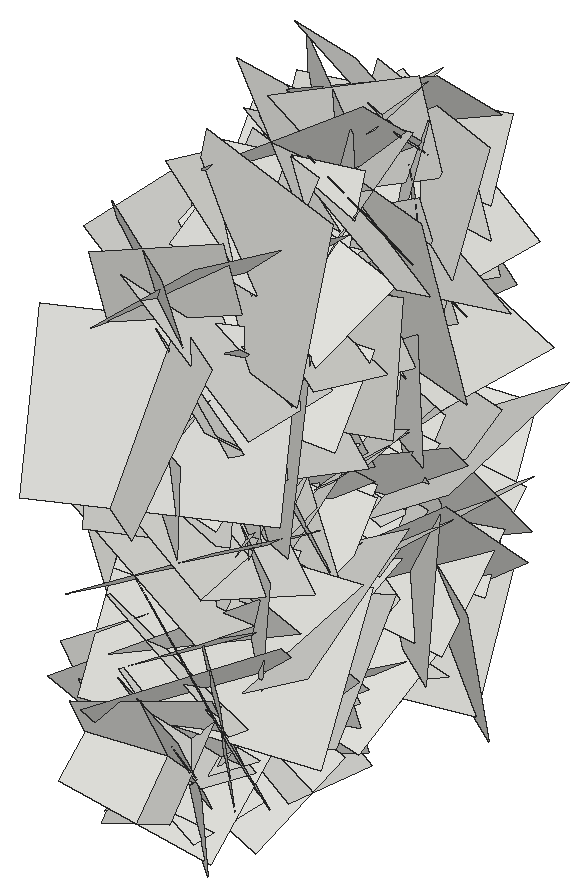
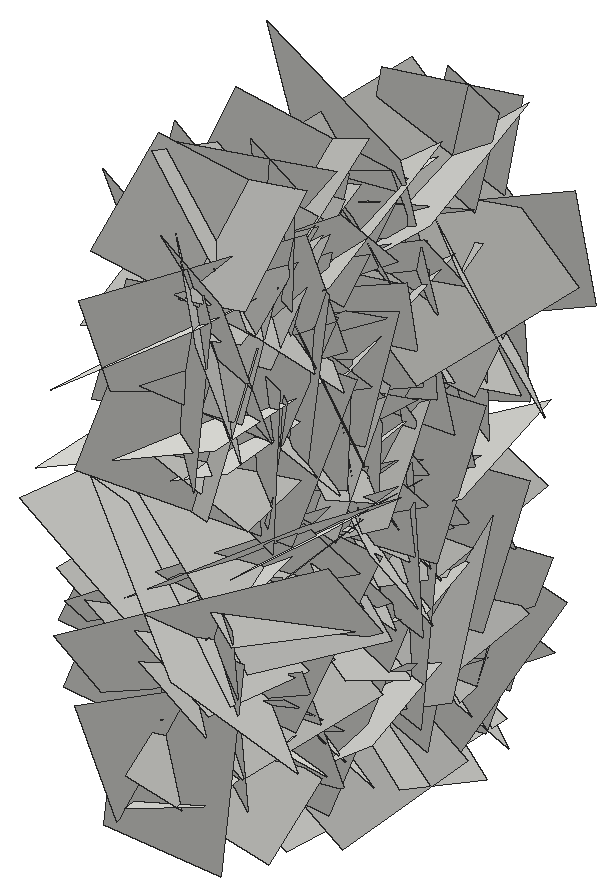
# SketchUp Ruby script. Lengths in inches.
U = 1.inch
M = Sketchup.active_model
def pt(a) = Geom::Point3d.new(a.map { |v| v * U })
def face(e, loops, mat)
  f = e.add_face(loops[0].map { |a| pt(a) })
  loops[1..].each { |l| e.add_face(l.map { |a| pt(a) }).erase! }
  f.material = f.back_material = mat if mat
  f
end
# faces: each face lists its corners as indices into pts; further lists are holes
def faces(e, pts, list, mat = nil) = list.each { |f| face(e, (f[0].is_a?(Array) ? f : [f]).map { |l| l.map { |i| pts[i] } }, mat) }
# xy, xz, yz: faces in a plane at the given z, y or x. An outline is a flat list of corners, or four numbers for a rectangle; further outlines are holes
def ring(l) = l.size == 4 ? [[l[0], l[1]], [l[2], l[1]], [l[2], l[3]], [l[0], l[3]]] : l.each_slice(2).to_a
def flat(e, list, mat, &to3) = list.each { |f| face(e, (f[0].is_a?(Array) ? f : [f]).map { |l| ring(l).map { |u, v| to3.(u, v) } }, mat) }
def xy(e, z, list, mat = nil) = flat(e, list, mat) { |x, y| [x, y, z] }
def xz(e, y, list, mat = nil) = flat(e, list, mat) { |x, z| [x, y, z] }
def yz(e, x, list, mat = nil) = flat(e, list, mat) { |y, z| [x, y, z] }
def lines(e, pts, list) = list.each { |a, b| e.add_line(pt(pts[a]), pt(pts[b])) }
# prism: a flat outline (further loops are holes) pulled along v
def prism(e, loops, v, mat = nil)
  f = face(e, loops, mat); d = Geom::Vector3d.new(v.map { |x| x * U })
  f.pushpull(f.normal.samedirection?(d) ? d.length : -d.length)
end
def box(e, o, s, mat = nil) = prism(e, [[o, [o[0] + s[0], o[1], o[2]], [o[0] + s[0], o[1] + s[1], o[2]], [o[0], o[1] + s[1], o[2]]]], [0, 0, s[2]], mat)
def at(x, y, z, deg = 0) = Geom::Transformation.translation(pt([x, y, z])) * Geom::Transformation.rotation(ORIGIN, Z_AXIS, deg.degrees)
def axes(o, x, y, z) = Geom::Transformation.new([*x, 0, *y, 0, *z, 0, *pt(o).to_a, 1])
def part(name) = M.definitions.add(name)
# library, detail: a bought-in or finely detailed component or shape, given as its bounding box
def library(name, o, s) = part(name).tap { |d| box(d.entities, o, s) }
def detail(e, o, s) = box(e.add_group.entities, o, s)
def put(e, d, t, mat = nil) = e.add_instance(d, t).tap { |i| i.material = mat if mat }
def group(e, t, mat = nil) = e.add_group.tap { |g| g.transformation = t; g.material = mat if mat }.entities
root = M.entities
c1 = part("Component\#6")
p = [[0.01,0,0],[0,3.24,4.54],[4.32,3.24,4.54],[4.33,0,0]]
faces(c1.entities,p,[[0,1,2,3]])
put(root,c1,axes([38.11,176.05,33.17],[-0.01986,0.50916,-0.88553],[0.06176,-0.8837,-0.50934],[-1.08099,-0.05984,-0.01283]))
put(root,c1,axes([38.11,182.77,28.15],[0.11013,-1.0722,-0.31704],[0.03816,-0.31503,1.07721],[-1.18456,-0.10983,0.00522]))
put(root,c1,axes([38.11,185.38,28.27],[0.28552,-0.8956,-0.93898],[0.07116,-0.9481,0.92355],[-1.37362,-0.23528,-0.14733]))
put(root,c1,axes([34.14,175.43,34.87],[-0.0411,0.62613,0.35799],[-0.03637,0.3565,-0.62724],[0.76365,0.05068,-0.01061]))
put(root,c1,axes([34.14,173.67,32.24],[-0.05341,-0.65994,-0.37026],[-0.06447,-0.36634,0.66124],[0.79951,-0.07362,0.02859]))
put(root,c1,axes([38.11,174.01,26.46],[0.07872,-0.97306,0.24072],[-0.0738,0.23579,0.97461],[-1.05998,-0.08868,-0.04998]))
put(root,c1,axes([38.11,170.16,39.2],[0.24703,1.2789,-0.21613],[0.13589,-0.24123,-1.28918],[-1.36812,0.20696,-0.16707]))
put(root,c1,axes([34.14,173.15,22.23],[0.01199,-0.5915,0.12784],[0.10227,0.12799,0.58366],[0.63327,-0.00947,-0.09668]))
put(root,c1,axes([38.11,167.34,31.77],[0.2501,0.51374,1.1242],[0.05799,1.13903,-0.532],[-1.3089,0.14863,0.19123]))
put(root,c1,axes([34.14,174.375,32.02],[-0.18574,0.64681,-0.5499],[-0.00393,-0.56207,-0.65994],[0.8999,0.13105,-0.11638]))
put(root,c1,axes([34.14,171.42,39.46],[0.01769,0.21401,-0.61924],[0.03571,-0.6189,-0.21298],[0.69357,0.02641,0.02676]))
put(root,c1,axes([34.14,180.11,41],[-0.0874,0.13713,-0.78202],[-0.02965,-0.78624,-0.13492],[0.84107,-0.01347,-0.08602]))
put(root,c1,axes([38.11,182.1,27.04],[0.18817,-1.1788,-0.21223],[0.10509,-0.19936,1.19019],[-1.26526,-0.19187,0.06729]))
put(root,c1,axes([38.11,177.13,31.79],[0.078,-0.30439,1.03044],[0.07955,1.03178,0.29943],[-1.13614,0.05135,0.09171]))
put(root,c1,axes([38.11,172.13,35.78],[-0.07615,0.65901,-0.5201],[-0.04859,-0.52431,-0.658],[-0.88857,-0.02781,0.08055]))
put(root,c1,axes([38.11,172.625,27.43],[0.01975,0.58315,0.74345],[-0.01761,0.74368,-0.58292],[-1.00141,-0.00157,0.02491]))
put(root,c1,axes([38.11,173.5,20.5],[0.29119,-0.77592,0.90535],[-0.00734,0.92801,0.79744],[-1.26387,-0.18415,0.20396]))
put(root,c1,axes([38.11,181.8125,37.17],[0.0246,-0.63961,0.56311],[-0.17949,0.54862,0.63013],[-0.88529,-0.129,-0.11211]))
put(root,c1,axes([34.14,177.7,39.03],[-0.08239,-0.33737,-0.64844],[0.10668,-0.65083,0.32654],[0.76743,0.05425,-0.11501]))
put(root,c1,axes([38.11,176.41,32.2],[-0.11408,-0.0942,-0.79779],[-0.0272,-0.8041,0.09841],[-0.85109,0.03832,0.10379]))
put(root,c1,axes([38.11,171.36,22.89],[-0.02535,0.88672,0.32576],[0.06435,0.32663,-0.88464],[-0.99927,-0.00146,-0.06523]))
put(root,c1,axes([38.11,178.05,19.9375],[0.14578,-1.0409,0.22357],[0.02192,0.228,1.04879],[-1.1283,-0.13006,0.04926]))
put(root,c1,axes([38.11,180.04,24.28],[-0.15161,0.71603,-0.23582],[-0.04269,-0.24694,-0.72538],[-0.79796,-0.12284,0.08362]))
put(root,c1,axes([34.14,173.29,20.87],[0.09428,-0.62013,-0.08152],[0.03551,-0.0775,0.6261],[0.66205,0.09247,-0.02197]))
put(root,c1,axes([34.14,173.36,27.66],[-0.12062,0.63946,0.63128],[-0.06443,0.62939,-0.6485],[0.9503,0.12384,0.03616]))
put(root,c1,axes([38.11,175.14,30.45],[0.22771,0.17317,-1.07869],[-0.0194,-1.09862,-0.18001],[-1.15789,0.05246,-0.20912]))
put(root,c1,axes([38.11,184.3,37.98],[0.01849,-0.42221,-1.00939],[0.24573,-0.98518,0.41609],[-1.13346,-0.22047,0.07374]))
put(root,c1,axes([34.14,172.01,32.68],[0.01531,-0.04852,-0.71126],[0.05574,-0.70939,0.04946],[0.75363,0.05345,0.01079]))
put(root,c1,axes([38.11,172,20.82],[0.19013,-0.4174,1.11707],[0.18593,1.12659,0.39279],[-1.25031,0.10406,0.22828]))
put(root,c1,axes([38.11,178.01,36.42],[-0.04909,-0.68925,0.58112],[0.09024,0.57594,0.68989],[-0.95135,0.0902,0.03545]))
put(root,c1,axes([38.11,174.95,31.63],[-0.12097,-0.07785,-0.70642],[-0.09105,-0.70871,0.09198],[-0.74781,0.09888,0.10307]))
put(root,c1,axes([34.14,171.52,27.71],[-0.03995,0.48298,0.66079],[-0.01207,0.66111,-0.48387],[0.8675,0.03144,0.0237]))
put(root,c1,axes([38.11,174.16,29.86],[-0.19319,0.59277,-0.26834],[-0.07097,-0.29428,-0.60458],[-0.68606,-0.13648,0.1381]))
put(root,c1,axes([38.11,171.18,26.98],[0.09963,0.88743,-0.23237],[-0.05305,-0.22828,-0.89204],[-0.97094,0.10354,0.02489]))
put(root,c1,axes([38.11,169.05,21.98],[-0.04882,0.58162,0.59704],[0.02934,0.59868,-0.58109],[-0.88303,-0.01226,-0.05232]))
put(root,c1,axes([38.11,176.26,32.94],[-0.03084,0.60524,0.59943],[0.03406,0.60013,-0.60439],[-0.90231,0.00196,-0.0433]))
put(root,c1,axes([38.11,174.875,32.24],[-0.12053,0.70886,0.38052],[0.08644,0.39248,-0.70676],[-0.84842,-0.06072,-0.12606]))
put(root,c1,axes([38.11,177.89,30.77],[-0.05678,-0.11721,0.8526],[0.09083,0.84928,0.12214],[-0.90772,0.09231,-0.04111]))
put(root,c1,axes([38.11,177.99,23.55],[-0.04107,0.5427,0.4395],[-0.20397,0.41484,-0.52921],[-0.71159,-0.15024,0.12632]))
put(root,c1,axes([38.11,174.67,32.54],[0.17055,0.3665,0.95024],[0.03456,0.95968,-0.37566],[-1.07902,0.08867,0.13816]))
put(root,c1,axes([38.11,176.52,27.27],[-0.06139,-0.83333,-0.30669],[0.14477,-0.31205,0.82208],[-0.93005,0.00643,0.1482]))
put(root,c1,axes([34.14,180.66,33.34],[-0.08177,-0.45253,0.73357],[0.03972,0.73405,0.45677],[0.91278,-0.07248,0.04584]))
put(root,c1,axes([34.14,181.67,36.78],[-0.05967,0.56874,-0.94691],[-0.29528,-0.9248,-0.5389],[1.13301,-0.21107,-0.19031]))
put(root,c1,axes([34.14,170.91,25.11],[0.00896,0.33986,-0.6335],[0.15678,-0.62081,-0.33108],[0.74574,0.12644,0.07722]))
put(root,c1,axes([38.11,182.09,31.375],[-0.0562,-0.72005,0.10613],[-0.07977,0.11126,0.71729],[-0.76737,0.04117,-0.08234]))
put(root,c1,axes([34.14,175.72,36.8],[-0.15665,0.75943,0.7145],[-0.11122,0.70715,-0.77331],[1.09966,0.17971,0.02357]))
put(root,c1,axes([38.11,175.72,36.8],[0.15665,0.75943,0.7145],[0.11122,0.70715,-0.77331],[-1.09966,0.17971,0.02357]))
put(root,c1,axes([34.14,182.09,31.375],[0.0562,-0.72005,0.10613],[0.07977,0.11126,0.71729],[0.76737,0.04117,-0.08234]))
put(root,c1,axes([38.11,170.91,25.11],[-0.00896,0.33986,-0.6335],[-0.15678,-0.62081,-0.33108],[-0.74574,0.12644,0.07722]))
put(root,c1,axes([38.11,181.67,36.78],[0.05967,0.56874,-0.94691],[0.29528,-0.9248,-0.5389],[-1.13301,-0.21107,-0.19031]))
put(root,c1,axes([38.11,180.66,33.34],[0.08177,-0.45253,0.73357],[-0.03972,0.73405,0.45677],[-0.91278,-0.07248,0.04584]))
put(root,c1,axes([34.14,176.52,27.27],[0.06139,-0.83333,-0.30669],[-0.14477,-0.31205,0.82208],[0.93005,0.00643,0.1482]))
put(root,c1,axes([34.14,174.67,32.54],[-0.17055,0.3665,0.95024],[-0.03456,0.95968,-0.37566],[1.07902,0.08867,0.13816]))
put(root,c1,axes([34.14,177.99,23.55],[0.04107,0.5427,0.4395],[0.20397,0.41484,-0.52921],[0.71159,-0.15024,0.12632]))
put(root,c1,axes([34.14,177.89,30.77],[0.05678,-0.11721,0.8526],[-0.09083,0.84928,0.12214],[0.90772,0.09231,-0.04111]))
put(root,c1,axes([34.14,174.875,32.24],[0.12053,0.70886,0.38052],[-0.08644,0.39248,-0.70676],[0.84842,-0.06072,-0.12606]))
put(root,c1,axes([34.14,176.26,32.94],[0.03084,0.60524,0.59943],[-0.03406,0.60013,-0.60439],[0.90231,0.00196,-0.0433]))
put(root,c1,axes([34.14,169.05,21.98],[0.04882,0.58162,0.59704],[-0.02934,0.59868,-0.58109],[0.88303,-0.01226,-0.05232]))
put(root,c1,axes([34.14,171.18,26.98],[-0.09963,0.88743,-0.23237],[0.05305,-0.22828,-0.89204],[0.97094,0.10354,0.02489]))
put(root,c1,axes([34.14,174.16,29.86],[0.19319,0.59277,-0.26834],[0.07097,-0.29428,-0.60458],[0.68606,-0.13648,0.1381]))
put(root,c1,axes([38.11,171.52,27.71],[0.03995,0.48298,0.66079],[0.01207,0.66111,-0.48387],[-0.8675,0.03144,0.0237]))
put(root,c1,axes([34.14,174.95,31.63],[0.12097,-0.07785,-0.70642],[0.09105,-0.70871,0.09198],[0.74781,0.09888,0.10307]))
put(root,c1,axes([34.14,178.01,36.42],[0.04909,-0.68925,0.58112],[-0.09024,0.57594,0.68989],[0.95135,0.0902,0.03545]))
put(root,c1,axes([34.14,172,20.82],[-0.19013,-0.4174,1.11707],[-0.18593,1.12659,0.39279],[1.25031,0.10406,0.22828]))
put(root,c1,axes([38.11,172.01,32.68],[-0.01531,-0.04852,-0.71126],[-0.05574,-0.70939,0.04946],[-0.75363,0.05345,0.01079]))
put(root,c1,axes([34.14,184.3,37.98],[-0.01849,-0.42221,-1.00939],[-0.24573,-0.98518,0.41609],[1.13346,-0.22047,0.07374]))
put(root,c1,axes([34.14,175.14,30.45],[-0.22771,0.17317,-1.07869],[0.0194,-1.09862,-0.18001],[1.15789,0.05246,-0.20912]))
put(root,c1,axes([38.11,173.36,27.66],[0.12062,0.63946,0.63128],[0.06443,0.62939,-0.6485],[-0.9503,0.12384,0.03616]))
put(root,c1,axes([38.11,173.29,20.87],[-0.09428,-0.62013,-0.08152],[-0.03551,-0.0775,0.6261],[-0.66205,0.09247,-0.02197]))
put(root,c1,axes([34.14,180.04,24.28],[0.15161,0.71603,-0.23582],[0.04269,-0.24694,-0.72538],[0.79796,-0.12284,0.08362]))
put(root,c1,axes([34.14,178.05,19.9375],[-0.14578,-1.0409,0.22357],[-0.02192,0.228,1.04879],[1.1283,-0.13006,0.04926]))
put(root,c1,axes([34.14,171.36,22.89],[0.02535,0.88672,0.32576],[-0.06435,0.32663,-0.88464],[0.99927,-0.00146,-0.06523]))
put(root,c1,axes([34.14,176.41,32.2],[0.11408,-0.0942,-0.79779],[0.0272,-0.8041,0.09841],[0.85109,0.03832,0.10379]))
put(root,c1,axes([38.11,177.7,39.03],[0.08239,-0.33737,-0.64844],[-0.10668,-0.65083,0.32654],[-0.76743,0.05425,-0.11501]))
put(root,c1,axes([34.14,181.8125,37.17],[-0.0246,-0.63961,0.56311],[0.17949,0.54862,0.63013],[0.88529,-0.129,-0.11211]))
put(root,c1,axes([34.14,173.5,20.5],[-0.29119,-0.77592,0.90535],[0.00734,0.92801,0.79744],[1.26387,-0.18415,0.20396]))
put(root,c1,axes([34.14,172.625,27.43],[-0.01975,0.58315,0.74345],[0.01761,0.74368,-0.58292],[1.00141,-0.00157,0.02491]))
put(root,c1,axes([34.14,172.13,35.78],[0.07615,0.65901,-0.5201],[0.04859,-0.52431,-0.658],[0.88857,-0.02781,0.08055]))
put(root,c1,axes([34.14,177.13,31.79],[-0.078,-0.30439,1.03044],[-0.07955,1.03178,0.29943],[1.13614,0.05135,0.09171]))
put(root,c1,axes([34.14,182.1,27.04],[-0.18817,-1.1788,-0.21223],[-0.10509,-0.19936,1.19019],[1.26526,-0.19187,0.06729]))
put(root,c1,axes([38.11,180.11,41],[0.0874,0.13713,-0.78202],[0.02965,-0.78624,-0.13492],[-0.84107,-0.01347,-0.08602]))
put(root,c1,axes([38.11,171.42,39.46],[-0.01769,0.21401,-0.61924],[-0.03571,-0.6189,-0.21298],[-0.69357,0.02641,0.02676]))
put(root,c1,axes([38.11,174.375,32.02],[0.18574,0.64681,-0.5499],[0.00393,-0.56207,-0.65994],[-0.8999,0.13105,-0.11638]))
put(root,c1,axes([34.14,167.34,31.77],[-0.2501,0.51374,1.1242],[-0.05799,1.13903,-0.532],[1.3089,0.14863,0.19123]))
put(root,c1,axes([38.11,173.15,22.23],[-0.01199,-0.5915,0.12784],[-0.10227,0.12799,0.58366],[-0.63327,-0.00947,-0.09668]))
put(root,c1,axes([34.14,170.16,39.2],[-0.24703,1.2789,-0.21613],[-0.13589,-0.24123,-1.28918],[1.36812,0.20696,-0.16707]))
put(root,c1,axes([34.14,174.01,26.46],[-0.07872,-0.97306,0.24072],[0.0738,0.23579,0.97461],[1.05998,-0.08868,-0.04998]))
put(root,c1,axes([38.11,173.67,32.24],[0.05341,-0.65994,-0.37026],[0.06447,-0.36634,0.66124],[-0.79951,-0.07362,0.02859]))
put(root,c1,axes([38.11,175.43,34.87],[0.0411,0.62613,0.35799],[0.03637,0.3565,-0.62724],[-0.76365,0.05068,-0.01061]))
put(root,c1,axes([34.14,185.38,28.27],[-0.28552,-0.8956,-0.93898],[-0.07116,-0.9481,0.92355],[1.37362,-0.23528,-0.14733]))
put(root,c1,axes([34.14,182.77,28.15],[-0.11013,-1.0722,-0.31704],[-0.03816,-0.31503,1.07721],[1.18456,-0.10983,0.00522]))
put(root,c1,axes([34.14,176.05,33.17],[0.01986,0.50916,-0.88553],[-0.06176,-0.8837,-0.50934],[1.08099,-0.05984,-0.01283]))
put(root,c1,axes([38.11,182.27,37.76],[0.22679,0.05489,-0.89691],[0.06736,-0.9206,-0.04118],[-0.95012,-0.05216,-0.217]))
put(root,c1,axes([34.14,174.9,23.69],[-0.06803,0.90477,0.33383],[0.16872,0.33992,-0.89067],[1.00823,0.00417,0.17157]))
put(root,c1,axes([38.11,173.11,21.9],[0.05319,-0.68826,0.19248],[0.04456,0.19546,0.68797],[-0.75624,-0.03689,0.05408]))
put(root,c1,axes([38.11,178.15,33.23],[-0.08938,-0.00525,-0.60269],[0.06829,-0.60515,-0.00374],[-0.63521,-0.06432,0.0844]))
put(root,c1,axes([38.11,176.44,21.6],[0.04345,0.60879,-0.00304],[-0.10651,0.00376,-0.60183],[-0.63647,0.04093,0.10051]))
put(root,c1,axes([34.14,183.67,38.38],[0.04708,0.10578,-1.15378],[-0.2342,-1.13267,-0.11235],[1.2056,-0.22416,0.02323]))
put(root,c1,axes([34.14,173.31,35.98],[-0.01252,1.07454,-0.37217],[-0.12805,-0.37127,-1.06811],[1.19858,-0.02844,-0.11799]))
put(root,c1,axes([34.14,174.78,20.26],[0.10048,-0.39109,0.79293],[0.10042,0.79738,0.38196],[0.93179,-0.04376,-0.12667]))
put(root,c1,axes([38.11,180.68,27.18],[0.06604,-0.60003,0.10008],[-0.10227,0.08959,0.59716],[-0.63666,-0.07663,-0.08554]))
put(root,c1,axes([38.11,170.73,19.61],[0.06378,-0.15247,0.68566],[0.07422,0.68605,0.14641],[-0.74085,0.05561,0.0737]))
put(root,c1,axes([34.14,178.01,21.81],[0.00864,0.40014,0.99077],[-0.02339,0.99065,-0.39991],[1.13239,0.01741,-0.01582]))
put(root,c1,axes([38.11,178.13,40.15],[0.04908,0.64392,0.19174],[0.08573,0.18545,-0.64234],[-0.70699,0.06719,-0.06458]))
put(root,c1,axes([34.14,171.95,33.74],[-0.07102,0.70639,0.8167],[0.11892,0.8184,-0.69866],[1.13841,-0.04142,0.12393]))
put(root,c1,axes([38.11,176.07,37.03],[0.15674,-0.62528,-0.09698],[-0.10666,-0.12156,0.63036],[-0.66219,-0.12843,-0.12449]))
put(root,c1,axes([38.11,180.42,25.12],[0.17902,-0.88337,-0.09354],[0.21931,-0.05348,0.8786],[-0.91571,-0.1855,0.19214]))
put(root,c1,axes([34.14,172.46,21.25],[0.14489,-0.73421,0.72244],[-0.08794,0.71856,0.74596],[1.0883,0.15581,-0.0359]))
put(root,c1,axes([34.14,171.47,32.36],[0.16942,0.96147,-0.31887],[-0.08969,-0.30901,-0.97416],[1.06999,-0.17814,-0.03117]))
put(root,c1,axes([34.14,179.35,38.14],[0.07028,1.07405,0.02302],[-0.04111,0.02544,-1.07534],[1.13802,-0.06541,-0.04027]))
put(root,c1,axes([38.11,181.39,28.46],[0.11732,-0.15238,-0.58962],[-0.01785,-0.59981,0.15186],[-0.64528,-0.01111,-0.1114]))
put(root,c1,axes([38.11,173.74,31.89],[0.15856,-0.67469,0.29232],[0.1064,0.31425,0.67394],[-0.77211,-0.09525,0.1529]))
put(root,c1,axes([34.14,173.84,39.64],[-0.13369,1.27699,-0.41872],[-0.11509,-0.42887,-1.27523],[1.41986,0.08547,-0.14279]))
put(root,c1,axes([38.11,172.58,29],[0.14706,-0.68518,0.03236],[0.10474,0.05263,0.69082],[-0.71951,-0.13238,0.10718]))
put(root,c1,axes([34.14,180.75,35.09],[-0.01445,0.08276,-1.11066],[0.1396,-1.10283,-0.0838],[1.17228,0.13235,-0.00371]))
put(root,c1,axes([34.14,182.25,27.43],[-0.1955,0.46825,-1.21407],[0.10064,-1.21809,-0.48422],[1.37564,0.15566,-0.13711]))
put(root,c1,axes([34.14,175.96,26.52],[0.03553,0.82214,0.9074],[-0.07429,0.90754,-0.81968],[1.2958,0.02948,-0.07187]))
put(root,c1,axes([34.14,172.47,36.95],[0.1233,0.89549,0.4145],[0.21728,0.38634,-0.89217],[1.02316,-0.18996,0.13951]))
put(root,c1,axes([34.14,183.25,38.77],[-0.07927,-0.40868,-1.12281],[0.1988,-1.11508,0.39337],[1.25087,0.15132,-0.13368]))
put(root,c1,axes([34.14,179.04,23.77],[0.11323,-0.75693,-0.7774],[0.09292,-0.77258,0.76428],[1.14637,0.13739,0.01483]))
put(root,c1,axes([34.14,182.77,28.7],[-0.0358,-0.11408,-1.31406],[-0.04325,-1.31377,0.1151],[1.39747,-0.04358,-0.0301]))
put(root,c1,axes([34.14,180.07,24.39],[-0.06666,-0.76105,0.92501],[0.21989,0.90537,0.75899],[1.25053,-0.19976,-0.08415]))
put(root,c1,axes([34.14,177.97,39.67],[-0.02985,0.75948,-0.84861],[0.27983,-0.8214,-0.74388],[1.17429,0.21504,0.15569]))
put(root,c1,axes([34.14,174.06,31.875],[0.08593,-0.00736,1.08266],[0.18405,1.07173,-0.00571],[1.1328,-0.17357,-0.0812]))
put(root,c1,axes([34.14,182.31,23.94],[-0.04872,-1.30982,0.04089],[0.01644,0.04037,1.31055],[1.38898,-0.04642,-0.01408]))
put(root,c1,axes([34.14,178.49,34.59],[0.00763,1.14917,-0.03145],[0.21412,-0.03223,-1.13128],[1.19962,-0.00155,0.20212]))
put(root,c1,axes([34.14,178.09,32.9],[0.18757,-0.47698,-1.21124],[-0.23196,-1.21588,0.44684],[1.36024,-0.14157,0.24323]))
put(root,c1,axes([34.14,178.68,21.25],[0.14964,-1.02559,0.91665],[-0.24358,0.89093,1.03221],[1.43757,0.25771,0.07948]))
put(root,c1,axes([34.14,169.91,24.28],[-0.0494,0.58776,1.07494],[0.25393,1.05932,-0.56884],[1.27358,-0.18841,0.15511]))
put(root,c1,axes([34.14,175.66,39.88],[-0.03914,-0.32872,-1.22009],[0.25418,-1.20026,0.31612],[1.31508,0.2222,-0.09741]))
put(root,c1,axes([34.14,177.96,25.04],[0.10915,-1.1796,-0.55067],[0.03689,-0.5497,1.18402],[1.37942,0.10803,0.01191]))
put(root,c1,axes([34.14,183.77,26.5],[0.0762,-1.33255,-0.21023],[0.04546,-0.20817,1.33413],[1.42926,0.07766,-0.03122]))
put(root,c1,axes([34.14,177.28,39.83],[0.04784,1.11638,-0.64936],[0.22797,-0.64718,-1.09769],[1.34988,0.06974,0.20839]))
put(root,c1,axes([34.14,179.625,37.91],[0.28026,0.12179,-1.29213],[0.26115,-1.29941,-0.07206],[1.35072,0.22596,0.28204]))
